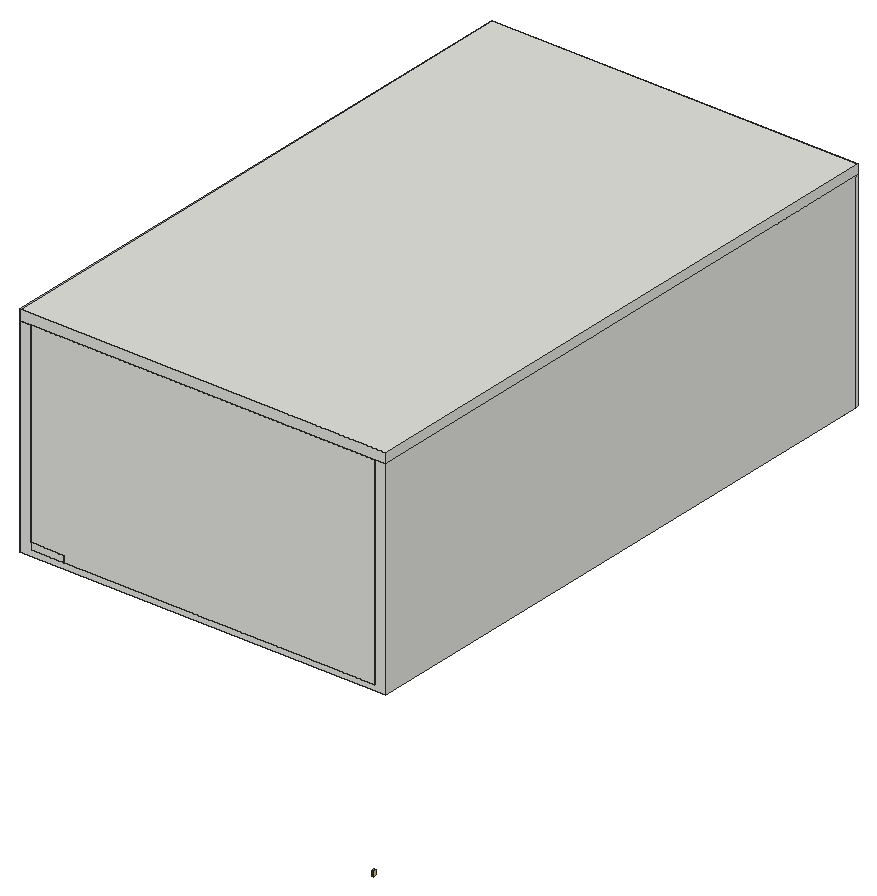
# SketchUp Ruby script. Lengths in inches.
U = 1.inch
M = Sketchup.active_model
def pt(a) = Geom::Point3d.new(a.map { |v| v * U })
def face(e, loops, mat)
  f = e.add_face(loops[0].map { |a| pt(a) })
  loops[1..].each { |l| e.add_face(l.map { |a| pt(a) }).erase! }
  f.material = f.back_material = mat if mat
  f
end
# faces: each face lists its corners as indices into pts; further lists are holes
def faces(e, pts, list, mat = nil) = list.each { |f| face(e, (f[0].is_a?(Array) ? f : [f]).map { |l| l.map { |i| pts[i] } }, mat) }
# xy, xz, yz: faces in a plane at the given z, y or x. An outline is a flat list of corners, or four numbers for a rectangle; further outlines are holes
def ring(l) = l.size == 4 ? [[l[0], l[1]], [l[2], l[1]], [l[2], l[3]], [l[0], l[3]]] : l.each_slice(2).to_a
def flat(e, list, mat, &to3) = list.each { |f| face(e, (f[0].is_a?(Array) ? f : [f]).map { |l| ring(l).map { |u, v| to3.(u, v) } }, mat) }
def xy(e, z, list, mat = nil) = flat(e, list, mat) { |x, y| [x, y, z] }
def xz(e, y, list, mat = nil) = flat(e, list, mat) { |x, z| [x, y, z] }
def yz(e, x, list, mat = nil) = flat(e, list, mat) { |y, z| [x, y, z] }
def lines(e, pts, list) = list.each { |a, b| e.add_line(pt(pts[a]), pt(pts[b])) }
# prism: a flat outline (further loops are holes) pulled along v
def prism(e, loops, v, mat = nil)
  f = face(e, loops, mat); d = Geom::Vector3d.new(v.map { |x| x * U })
  f.pushpull(f.normal.samedirection?(d) ? d.length : -d.length)
end
def box(e, o, s, mat = nil) = prism(e, [[o, [o[0] + s[0], o[1], o[2]], [o[0] + s[0], o[1] + s[1], o[2]], [o[0], o[1] + s[1], o[2]]]], [0, 0, s[2]], mat)
def at(x, y, z, deg = 0) = Geom::Transformation.translation(pt([x, y, z])) * Geom::Transformation.rotation(ORIGIN, Z_AXIS, deg.degrees)
def axes(o, x, y, z) = Geom::Transformation.new([*x, 0, *y, 0, *z, 0, *pt(o).to_a, 1])
def part(name) = M.definitions.add(name)
# library, detail: a bought-in or finely detailed component or shape, given as its bounding box
def library(name, o, s) = part(name).tap { |d| box(d.entities, o, s) }
def detail(e, o, s) = box(e.add_group.entities, o, s)
def put(e, d, t, mat = nil) = e.add_instance(d, t).tap { |i| i.material = mat if mat }
def group(e, t, mat = nil) = e.add_group.tap { |g| g.transformation = t; g.material = mat if mat }.entities
root = M.entities
M.materials.add("Material__1").color = [189, 132, 57]
M.materials.add("Material__10").color = [180, 24, 1]
M.materials.add("Material__2").color = [242, 239, 230]
M.materials.add("Material__3").color = [122, 114, 11]
M.materials.add("[0005_LightPink]").color = [206, 147, 156]
M.materials.add("[0007_MistyRose]").color = [255, 228, 225]
M.materials.add("[0011_Seashell]").color = [242, 232, 226]
M.materials.add("[0012_Bisque]").color = [255, 228, 196]
M.materials.add("[0021_DarkRed]").color = [58, 0, 0]
M.materials.add("[0022_Maroon]").color = [58, 0, 0]
M.materials.add("[0030_OldLace]").color = [253, 245, 230]
M.materials.add("[Color_000]").color = [255, 255, 255]
M.materials.add("[Color_004]").color = [142, 142, 142]
M.materials.add("[Tile Large Brown]").color = [193, 176, 158]
M.materials.add("cnwhc.com_草图联盟_1kmauOsh").color = [54, 52, 52]
M.materials.add("cnwhc.com_草图联盟_C8Y5Xp2O").color = [156, 156, 156]
M.materials["cnwhc.com_草图联盟_C8Y5Xp2O"].alpha = 0.15
M.materials.add("cnwhc.com_草图联盟_IHFcDxe1").color = [138, 151, 59]
M.materials.add("cnwhc.com_草图联盟_KNEfX85g").color = [162, 126, 87]
M.materials.add("cnwhc.com_草图联盟_QJow1Ky4").color = [144, 133, 65]
M.materials.add("cnwhc.com_草图联盟_z6N5x4Hv").color = [223, 205, 124]
c1 = library("JD\#1",[0,0,0],[1.32,0.83,0.01])
c2 = part("Untitled (20)")
xy(c2.entities,0,[[0,0,43.31,7.875],[43.31,0,47.24,7.875]],"[Color_000]")
xy(c2.entities,1.97,[[3.9375,0,43.31,3.15],[3.9375,3.15,23.62,4.72],[23.62,3.15,43.31,4.72],[3.9375,4.72,43.31,7.875]],"[Color_000]")
xy(c2.entities,3.9375,[[5.91,3.15,21.65,3.9375],[25.59,3.15,41.34,3.9375],[5.91,3.9375,21.65,4.72],[25.59,3.9375,41.34,4.72]],"[Color_000]")
xy(c2.entities,17.81,[[5.91,3.15,21.65,3.9375],[25.59,3.15,41.34,3.9375],[5.91,3.9375,21.65,4.72],[25.59,3.9375,41.34,4.72]],"[Color_000]")
xy(c2.entities,18.6,[[5.91,3.15,21.65,3.9375],[25.59,3.15,41.34,3.9375],[5.91,3.9375,21.65,4.72],[25.59,3.9375,41.34,4.72]],"[Color_000]")
xy(c2.entities,28.25,[[22.3,4.72,22.85,5.91],[24.27,4.72,24.8125,5.91]],"[Color_004]")
xy(c2.entities,29.04,[[22.3,4.72,22.85,5.51],[24.27,4.72,24.8125,5.51]],"[Color_004]")
xy(c2.entities,32.09,[[5.91,3.15,21.65,3.9375],[25.59,3.15,41.34,3.9375],[5.91,3.9375,21.65,4.72],[25.59,3.9375,41.34,4.72]],"[Color_000]")
xy(c2.entities,32.875,[[5.91,3.15,21.65,3.9375],[25.59,3.15,41.34,3.9375],[5.91,3.9375,21.65,4.72],[25.59,3.9375,41.34,4.72]],"[Color_000]")
xy(c2.entities,35.79,[[22.3,4.72,22.85,5.51],[24.27,4.72,24.8125,5.51]],"[Color_004]")
xy(c2.entities,36.58,[[22.3,4.72,22.85,5.91],[24.27,4.72,24.8125,5.91]],"[Color_004]")
xy(c2.entities,46.36,[[5.91,3.15,21.65,3.9375],[25.59,3.15,41.34,3.9375],[5.91,3.9375,21.65,4.72],[25.59,3.9375,41.34,4.72]],"[Color_000]")
xy(c2.entities,47.15,[[5.91,3.15,21.65,3.9375],[25.59,3.15,41.34,3.9375],[5.91,3.9375,21.65,4.72],[25.59,3.9375,41.34,4.72]],"[Color_000]")
xy(c2.entities,61.02,[[5.91,3.15,21.65,3.9375],[25.59,3.15,41.34,3.9375],[5.91,3.9375,21.65,4.72],[25.59,3.9375,41.34,4.72]],"[Color_000]")
xy(c2.entities,62.99,[[3.9375,0,43.31,3.15],[3.9375,3.15,23.62,4.72],[23.62,3.15,43.31,4.72],[3.9375,4.72,43.31,7.875]],"[Color_000]")
xy(c2.entities,66.93,[[0,0,47.24,7.875]],"[Color_000]")
xz(c2.entities,0,[[0,0,0,66.93,47.24,66.93,47.24,0,43.31,0,43.31,62.99,3.9375,62.99,3.9375,0],[3.9375,0,43.31,1.97]],"[Color_000]")
xz(c2.entities,3.15,[[[3.9375,1.97,23.62,62.99],[5.91,47.15,21.65,61.02],[5.91,3.9375,21.65,17.81],[5.91,18.6,21.65,32.09],[5.91,32.875,21.65,46.36]],[[23.62,1.97,43.31,62.99],[25.59,3.9375,41.34,17.81],[25.59,47.15,41.34,61.02],[25.59,18.6,41.34,32.09],[25.59,32.875,41.34,46.36]]],"[Color_000]")
xz(c2.entities,3.9375,[[5.91,3.9375,21.65,17.81],[25.59,3.9375,41.34,17.81],[5.91,18.6,21.65,32.09],[25.59,18.6,41.34,32.09],[5.91,32.875,21.65,46.36],
  [25.59,32.875,41.34,46.36],[5.91,47.15,21.65,61.02],[25.59,47.15,41.34,61.02]])
xz(c2.entities,4.72,[[[3.9375,1.97,23.62,62.99],[5.91,3.9375,21.65,17.81],[5.91,47.15,21.65,61.02],[5.91,18.6,21.65,32.09],[5.91,32.875,21.65,46.36]],[[23.62,1.97,43.31,62.99],[25.59,3.9375,41.34,17.81],[25.59,47.15,41.34,61.02],[25.59,18.6,41.34,32.09],[25.59,32.875,41.34,46.36]]],"[Color_000]")
xz(c2.entities,5.51,[[22.3,29.04,22.85,35.79],[24.27,29.04,24.8125,35.79]],"[Color_004]")
xz(c2.entities,5.91,[[22.3,28.25,22.85,36.58],[24.27,28.25,24.8125,36.58]],"[Color_004]")
xz(c2.entities,7.875,[[0,0,3.9375,0,3.9375,62.99,43.31,62.99,43.31,0,47.24,0,47.24,66.93,0,66.93],[3.9375,0,43.31,1.97]],"[Color_000]")
yz(c2.entities,0,[[0,0,7.875,66.93]],"[Color_000]")
yz(c2.entities,3.9375,[[0,1.97,3.15,62.99],[3.15,1.97,4.72,62.99],[4.72,1.97,7.875,62.99]],"[Color_000]")
yz(c2.entities,5.91,[[3.15,3.9375,3.9375,17.81],[3.9375,3.9375,4.72,17.81],[3.15,18.6,3.9375,32.09],[3.9375,18.6,4.72,32.09],[3.15,32.875,3.9375,46.36],
  [3.9375,32.875,4.72,46.36],[3.15,47.15,3.9375,61.02],[3.9375,47.15,4.72,61.02]],"[Color_000]")
yz(c2.entities,21.65,[[3.15,3.9375,3.9375,17.81],[3.9375,3.9375,4.72,17.81],[3.15,18.6,3.9375,32.09],[3.9375,18.6,4.72,32.09],[3.15,32.875,3.9375,46.36],
  [3.9375,32.875,4.72,46.36],[3.15,47.15,3.9375,61.02],[3.9375,47.15,4.72,61.02]],"[Color_000]")
yz(c2.entities,22.3,[[4.72,28.25,4.72,29.04,5.51,29.04,5.51,35.79,4.72,35.79,4.72,36.58,5.91,36.58,5.91,28.25]],"[Color_004]")
yz(c2.entities,22.85,[[4.72,28.25,5.91,28.25,5.91,36.58,4.72,36.58,4.72,35.79,5.51,35.79,5.51,29.04,4.72,29.04]],"[Color_004]")
yz(c2.entities,23.62,[[3.15,1.97,4.72,62.99]],"[Color_000]")
yz(c2.entities,24.27,[[4.72,28.25,4.72,29.04,5.51,29.04,5.51,35.79,4.72,35.79,4.72,36.58,5.91,36.58,5.91,28.25]],"[Color_004]")
yz(c2.entities,24.8125,[[4.72,28.25,5.91,28.25,5.91,36.58,4.72,36.58,4.72,35.79,5.51,35.79,5.51,29.04,4.72,29.04]],"[Color_004]")
yz(c2.entities,25.59,[[3.15,3.9375,3.9375,17.81],[3.9375,3.9375,4.72,17.81],[3.15,18.6,3.9375,32.09],[3.9375,18.6,4.72,32.09],[3.15,32.875,3.9375,46.36],
  [3.9375,32.875,4.72,46.36],[3.15,47.15,3.9375,61.02],[3.9375,47.15,4.72,61.02]],"[Color_000]")
yz(c2.entities,41.34,[[3.15,3.9375,3.9375,17.81],[3.9375,3.9375,4.72,17.81],[3.15,18.6,3.9375,32.09],[3.9375,18.6,4.72,32.09],[3.15,32.875,3.9375,46.36],
  [3.9375,32.875,4.72,46.36],[3.15,47.15,3.9375,61.02],[3.9375,47.15,4.72,61.02]],"[Color_000]")
yz(c2.entities,43.31,[[0,0,7.875,1.97],[0,1.97,3.15,62.99],[3.15,1.97,4.72,62.99],[4.72,1.97,7.875,62.99]],"[Color_000]")
yz(c2.entities,47.24,[[0,0,7.875,66.93]],"[Color_000]")
put(c2.entities,c1,axes([39.54,3.9375,4.43],[1,0,0],[0,0,1],[0,-1,0]))
put(c2.entities,c1,axes([19.85,3.9375,4.43],[1,0,0],[0,0,1],[0,-1,0]))
c3 = library("B36CD50SNS_tradeCAD",[0,0,0],[35.84,30.35,69.65])
c4 = library("Oven",[-9.26,-22.59,0.07],[23.42,23.91,23.21])
c5 = library("ZSA1202RSS",[0,0,0],[29.9375,17.9,16.4375])
c6 = library("switch+board",[0,0,0],[0.88,10.49,5.27])
c7 = library("Grupo3\#1",[-2.41,-4.18,0],[4.82,8.16,14.49])
c8 = library("Group\#35",[-453.95,-270.9,-0.08],[243.89,243.63,216.82])
c9 = library("Group\#42",[118.34,-437.05,68.8],[33.09,42.97,27.32])
c10 = library("Group\#43",[91.875,-459.8125,1.36],[84.84,84.82,167.94])
c11 = library("Group\#44",[93.63,-458.06,3.28],[81.33,81.31,90.04])
c12 = library("Group\#45",[114.46,-437.1875,150.05],[39.68,39.57,39.67])
c13 = library("Group\#46",[177.52,-496.26,3.28],[81.21,81.23,127.94])
c14 = library("Group\#47",[175.77,-498.01,1.36],[84.71,84.74,167.94])
c15 = library("Group\#48",[198.24,-475.92,149.53],[39.78,40.55,40.71])
c16 = library("Group\#49",[-248.47,-468.28,0.39],[392.05,393.05,278.56])
c17 = library("Group\#50",[-141.57,-278.65,11.2],[96.36,96.33,131.41])
c18 = library("Group\#51",[-62.08,-202.43,11.2],[96.04,96.07,131.41])
c19 = library("Group\#52",[18.13,-280.93,11.2],[96.51,96.54,131.41])
c20 = library("Group\#53",[-213.25,-366.61,11.2],[96.18,96.15,131.41])
c21 = library("Group\#54",[-61.03,-358.93,11.2],[96.54,96.51,131.41])
c22 = library("Group\#55",[8.05,-292.87,22.71],[116.19,111.01,218.49])
c23 = library("Group\#56",[-64.85,-368.89,23],[127.95,108.9,222.0625])
c24 = library("Group\#57",[-143.92,-281.53,22.82],[119.68,105.06,218.38])
c25 = library("Group\#58",[-64.19,-232.55,22.9],[102.65,128.29,224.14])
c26 = library("Group\#59",[-225.25,-376.69,19.19],[116.52,116.69,261.73])
c27 = library("Group\#60",[-138.35,-437.94,11.2],[96.49,96.52,131.41])
c28 = library("Group\#61",[-142.58,-458.38,19.87],[79.66,135.74,256])
c29 = part("KITCHEN+ITEMS+(37)")
put(c29.entities,c8,at(0,0,0))
put(c29.entities,c9,at(0,0,0),"cnwhc.com_草图联盟_IHFcDxe1")
put(c29.entities,c10,at(0,0,0),"cnwhc.com_草图联盟_C8Y5Xp2O")
put(c29.entities,c11,at(0,0,0),"cnwhc.com_草图联盟_QJow1Ky4")
put(c29.entities,c12,at(0,0,0),"cnwhc.com_草图联盟_KNEfX85g")
put(c29.entities,c13,at(0,0,0),"cnwhc.com_草图联盟_z6N5x4Hv")
put(c29.entities,c14,at(0,0,0),"cnwhc.com_草图联盟_C8Y5Xp2O")
put(c29.entities,c15,at(0,0,0),"cnwhc.com_草图联盟_KNEfX85g")
put(c29.entities,c16,at(0,0,0),"cnwhc.com_草图联盟_1kmauOsh")
put(c29.entities,c17,at(0,0,0),"cnwhc.com_草图联盟_C8Y5Xp2O")
put(c29.entities,c18,at(0,0,0),"cnwhc.com_草图联盟_C8Y5Xp2O")
put(c29.entities,c19,at(0,0,0),"cnwhc.com_草图联盟_C8Y5Xp2O")
put(c29.entities,c20,at(0,0,0),"cnwhc.com_草图联盟_C8Y5Xp2O")
put(c29.entities,c21,at(0,0,0),"cnwhc.com_草图联盟_C8Y5Xp2O")
put(c29.entities,c22,at(0,0,0),"cnwhc.com_草图联盟_1kmauOsh")
put(c29.entities,c23,at(0,0,0),"cnwhc.com_草图联盟_1kmauOsh")
put(c29.entities,c24,at(0,0,0),"cnwhc.com_草图联盟_1kmauOsh")
put(c29.entities,c25,at(0,0,0),"cnwhc.com_草图联盟_1kmauOsh")
put(c29.entities,c26,at(0,0,0))
put(c29.entities,c27,at(0,0,0),"cnwhc.com_草图联盟_C8Y5Xp2O")
put(c29.entities,c28,at(0,0,0))
c30 = library("C_HOB",[0,0,0],[30.71,17.32,2.28])
c31 = library("Component_12",[0,0,0],[17.72,31.5,20.63])
c32 = library("secto_design_octo_lamp_150sm",[-45.69,-78.93,-193.9375],[1.18,1.52,2.78])
c33 = library("Untitled",[-2.37,-2.84,0],[34.77,46.37,39.61])
c34 = library("Group\#13",[70.57,7290.35,1177],[106.36,95.58,107.8])
c35 = library("Group\#14",[99.22,7286.02,1075.87],[101.63,96.21,134.31])
c36 = library("Group\#12",[73.8125,7223.02,1078.11],[130.55,102.07,69.6])
c37 = library("Group\#11",[51.66,7209.26,1075.25],[220.83,167.48,13.5625])
c38 = library("Group\#15",[141.6875,7219.59,1077.95],[111.05,77.92,100.97])
c39 = library("Group\#16",[180.93,7251.18,1124.56],[65.88,104.93,74.66])
c40 = library("Group\#39",[0,0,0],[35.16,49.83,62.5625])
xy(root,0,[[1.875,0,219.125,349.0625],[1.875,349.0625,219.125,350.4375]])
xy(root,3.25,[[27.875,0,212.75,0,212.75,344.4375,174.95,344.4375,174.95,324.4375,27.875,324.4375]],"[Tile Large Brown]")
xy(root,5.25,[[120.66,320.4375,121.78,324.4375],[174.04,320.4375,174.95,324.4375],[121.78,324.4375,174.04,342.4375]])
xy(root,7.25,[[7.875,0,27.875,206.4375],[7.875,206.4375,27.875,344.4375],[27.875,206.4375,27.875,324.4375,31.875,324.4375,31.875,305.07,31.75,305.07,31.75,304.77,31.875,304.77,31.875,285.4,31.75,285.4,31.75,285.1,31.875,285.1,31.875,265.74,31.57,265.74,31.57,265.4375,31.875,265.4375,31.875,246.07,31.57,246.07,31.57,245.77,31.875,245.77,31.875,226.4,31.57,226.4,31.57,226.1,31.875,226.1,31.875,206.4375],[31.875,320.4375,92.74,324.4375],[92.74,320.4375,120.66,324.4375],
  [27.875,324.4375,31.875,344.4375],[31.875,324.4375,92.74,344.4375]])
xy(root,21.0625,[[12.6,212.83,26.79,237.4]])
xy(root,23.61,[[94.18,320.4375,119.93,342.4375]])
xy(root,30.1875,[[[7.875,206.4375,7.875,344.4375,31.875,344.4375,31.875,305.07,31.75,305.07,31.75,304.77,31.875,304.77,31.875,285.4,31.75,285.4,31.75,285.1,31.875,285.1,31.875,265.74,31.57,265.74,31.57,265.4375,31.875,265.4375,31.875,246.07,31.57,246.07,31.57,245.77,31.875,245.77,31.875,226.4,31.57,226.4,31.57,226.1,31.875,226.1,31.875,206.4375],[12.6,212.83,26.79,237.4]],[31.875,320.4375,92.74,344.4375]])
xy(root,31.25,[[[7.875,206.4375,31.875,206.4375,31.875,226.1,31.57,226.1,31.57,226.4,31.875,226.4,31.875,245.77,31.57,245.77,31.57,246.07,31.875,246.07,31.875,265.4375,31.57,265.4375,31.57,265.74,31.875,265.74,31.875,285.1,31.75,285.1,31.75,285.4,31.875,285.4,31.875,304.77,31.75,304.77,31.75,305.07,31.875,305.07,31.875,344.4375,7.875,344.4375],[12.6,212.83,26.79,237.4]],[31.875,320.4375,92.74,344.4375]])
xy(root,39.25,[[1.875,241.12,7.875,291.68]])
xy(root,43.3,[[94.18,320.4375,119.93,342.4375]])
xy(root,43.97,[[94.18,320.4375,119.93,342.4375]])
xy(root,54.5,[[7.875,291.68,7.875,344.4375,92.74,344.4375,92.74,324.4375,68.82,324.4375,68.82,324.875,68.52,324.875,68.52,324.4375,48.35,324.4375,48.35,324.875,48.05,324.875,48.05,324.4375,27.875,324.4375,27.875,291.68]])
xy(root,55.25,[[7.875,291.68,27.875,291.68,27.875,324.4375,48.05,324.4375,48.05,324.875,48.35,324.875,48.35,324.4375,68.52,324.4375,68.52,324.875,68.82,324.875,68.82,324.4375,92.74,324.4375,92.74,344.4375,7.875,344.4375]])
xy(root,55.84,[[7.875,292.27,27.875,310.77]])
xy(root,56.48,[[94.18,320.4375,119.93,342.4375]])
xy(root,56.96,[[93.75,320.4375,120.66,320.5625]])
xy(root,57.46,[[94.25,320.4375,120.16,320.5625]])
xy(root,64.125,[[121.78,320.4375,147.91,342.4375],[147.91,320.4375,148.29,342.4375],[148.29,320.4375,172.91,342.4375],[172.91,320.4375,174.04,342.4375]])
xy(root,64.4375,[[121.78,320.4375,147.91,320.5625],[147.91,320.4375,148.29,320.5625],[148.29,320.4375,172.91,320.5625],[172.91,320.4375,174.04,320.5625]])
xy(root,64.71,[[122.0625,320.4375,147.63,320.5625],[148.5625,320.4375,172.91,320.5625],[172.91,320.4375,173.76,320.5625]])
xy(root,66.96,[[7.875,292.27,27.875,310.77]])
xy(root,67.65,[[7.875,292.27,27.875,310.77]])
xy(root,77.82,[[94.25,320.4375,120.16,320.5625]])
xy(root,78.04,[[122.0625,320.4375,147.63,320.5625],[148.5625,320.4375,173.76,320.5625]])
xy(root,78.09,[[7.875,292.27,27.875,310.77]])
xy(root,78.3125,[[93.75,320.4375,120.66,320.5625],[121.78,320.4375,147.91,320.5625],[147.91,320.4375,148.29,320.5625],[148.29,320.4375,174.04,320.5625]])
xy(root,78.75,[[7.875,291.68,27.875,318.0625],[7.875,318.0625,27.875,324.4375],[92.74,320.4375,174.95,320.4375,174.95,344.4375,169.83,344.4375,169.83,324.4375,149.85,324.4375,149.85,324.5625,149.55,324.5625,149.55,324.4375,129.57,324.4375,129.57,324.5625,129.27,324.5625,129.27,324.4375,109.29,324.4375,109.29,324.5625,108.99,324.5625,108.99,324.4375,92.74,324.4375],[7.875,324.4375,27.875,344.4375],[27.875,324.4375,36.16,344.4375],
  [36.16,324.4375,36.16,344.4375,64.45,344.4375,64.45,324.4375,48.35,324.4375,48.35,324.875,48.05,324.875,48.05,324.4375],[48.05,324.4375,48.35,324.875],[64.45,324.4375,64.45,344.4375,92.74,344.4375,92.74,324.4375,68.82,324.4375,68.82,324.875,68.52,324.875,68.52,324.4375],[68.52,324.4375,68.82,324.875]])
xy(root,78.75,[[7.875,206.4375,27.875,291.68]],"[0007_MistyRose]")
xy(root,79.25,[[7.875,206.4375,27.875,206.4375,27.875,226.1,27.75,226.1,27.75,226.4,27.875,226.4,27.875,241.12,7.875,241.12],[27.75,226.1,27.875,226.4],[1.875,241.12,7.875,291.68],[7.875,241.12,27.875,241.12,27.875,245.77,27.75,245.77,27.75,246.07,27.875,246.07,27.875,265.4375,27.75,265.4375,27.75,265.74,27.875,265.74,27.875,285.1,27.75,285.1,27.75,285.4,27.875,285.4,27.875,291.68,7.875,291.68],[27.75,245.77,27.875,246.07],
  [27.75,265.4375,27.875,265.74],[27.75,285.1,27.875,285.4],[7.875,291.68,27.875,291.68,27.875,304.77,27.75,304.77,27.75,305.07,27.875,305.07,27.875,324.4375,7.875,324.4375],[27.75,304.77,27.875,305.07],[7.875,324.4375,48.15,324.4375,48.15,324.5625,48.45,324.5625,48.45,324.4375,68.43,324.4375,68.43,324.5625,68.73,324.5625,68.73,324.4375,88.71,324.4375,88.71,324.5625,89.01,324.5625,89.01,324.4375,92.74,324.4375,92.74,344.4375,7.875,344.4375],
  [48.15,324.4375,48.45,324.5625],[68.43,324.4375,68.73,324.5625],[88.71,324.4375,89.01,324.5625],[92.74,324.4375,92.74,344.4375,169.83,344.4375,169.83,324.4375,149.85,324.4375,149.85,324.5625,149.55,324.5625,149.55,324.4375,129.57,324.4375,129.57,324.5625,129.27,324.5625,129.27,324.4375,109.29,324.4375,109.29,324.5625,108.99,324.5625,108.99,324.4375]])
xy(root,123.25,[[1.875,0,1.875,349.0625,219.125,349.0625,219.125,0,212.75,0,212.75,344.4375,7.875,344.4375,7.875,0],[7.875,0,27.875,206.4375],[7.875,206.4375,7.875,324.4375,27.875,324.4375,27.875,305.07,27.75,305.07,27.75,304.77,27.875,304.77,27.875,285.4,27.75,285.4,27.75,285.1,27.875,285.1,27.875,265.74,27.75,265.74,27.75,265.4375,27.875,265.4375,27.875,246.07,27.75,246.07,27.75,245.77,27.875,245.77,27.875,226.4,27.75,226.4,27.75,226.1,27.875,226.1,27.875,206.4375],[7.875,324.4375,7.875,344.4375,169.83,344.4375,169.83,324.4375,149.85,324.4375,149.85,324.5625,149.55,324.5625,149.55,324.4375,129.57,324.4375,129.57,324.5625,129.27,324.5625,129.27,324.4375,109.29,324.4375,109.29,324.5625,108.99,324.5625,108.99,324.4375,89.01,324.4375,89.01,324.5625,88.71,324.5625,88.71,324.4375,68.73,324.4375,68.73,324.5625,68.43,324.5625,68.43,324.4375,48.45,324.4375,48.45,324.5625,48.15,324.5625,48.15,324.4375],[1.875,349.0625,219.125,350.4375]])
xy(root,123.25,[[[95.39,234.92,146.73,296.17],[123.59,242.42,125.03,242.53,126.45,242.79,127.84,243.2,129.17,243.75,130.44,244.44,131.64,245.26,132.74,246.2,133.73,247.25,134.61,248.39,135.37,249.625,135.99,250.93,136.48,252.29,136.8125,253.7,137,255.13,137.04,256.58,136.93,258.02,136.67,259.4375,136.26,260.83,135.71,262.16,135.02,263.43,134.2,264.625,133.26,265.73,132.21,266.72,131.07,267.6,129.83,268.36,128.53,268.98,127.17,269.46,125.76,269.8,124.33,269.99,122.88,270.03,121.44,269.92,120.02,269.66,118.63,269.25,117.3,268.69,116.03,268.01,114.83,267.1875,113.73,266.25,112.74,265.2,111.86,264.05,111.1,262.82,110.48,261.52,109.99,260.15,109.65,258.75,109.47,257.32,109.43,255.87,109.54,254.43,109.8,253.01,110.21,251.62,110.76,250.29,111.45,249.01,112.27,247.82,113.21,246.72,114.26,245.73,115.4,244.85,116.64,244.09,117.94,243.47,119.3,242.98,120.71,242.64,122.14,242.45]]],"[0005_LightPink]")
xy(root,123.25,[[123.59,242.42,122.14,242.45,120.71,242.64,119.3,242.98,117.94,243.47,116.64,244.09,115.4,244.85,114.26,245.73,113.21,246.72,112.27,247.82,111.45,249.01,110.76,250.29,110.21,251.62,109.8,253.01,109.54,254.43,109.43,255.87,109.47,257.32,109.65,258.75,109.99,260.15,110.48,261.52,111.1,262.82,111.86,264.05,112.74,265.2,113.73,266.25,114.83,267.1875,116.03,268.01,117.3,268.69,118.63,269.25,120.02,269.66,121.44,269.92,122.88,270.03,124.33,269.99,125.76,269.8,127.17,269.46,128.53,268.98,129.83,268.36,131.07,267.6,132.21,266.72,133.26,265.73,134.2,264.625,135.02,263.43,135.71,262.16,136.26,260.83,136.67,259.4375,136.93,258.02,137.04,256.58,137,255.13,136.8125,253.7,136.48,252.29,135.99,250.93,135.37,249.625,134.61,248.39,133.73,247.25,132.74,246.2,131.64,245.26,130.44,244.44,129.17,243.75,127.84,243.2,126.45,242.79,125.03,242.53]],"[0022_Maroon]")
xy(root,123.25,[[[27.875,0,27.875,226.1,27.75,226.1,27.75,226.4,27.875,226.4,27.875,245.77,27.75,245.77,27.75,246.07,27.875,246.07,27.875,265.4375,27.75,265.4375,27.75,265.74,27.875,265.74,27.875,285.1,27.75,285.1,27.75,285.4,27.875,285.4,27.875,304.77,27.75,304.77,27.75,305.07,27.875,305.07,27.875,324.4375,48.15,324.4375,48.15,324.5625,48.45,324.5625,48.45,324.4375,68.43,324.4375,68.43,324.5625,68.73,324.5625,68.73,324.4375,88.71,324.4375,88.71,324.5625,89.01,324.5625,89.01,324.4375,108.99,324.4375,108.99,324.5625,109.29,324.5625,109.29,324.4375,129.27,324.4375,129.27,324.5625,129.57,324.5625,129.57,324.4375,149.55,324.4375,149.55,324.5625,149.85,324.5625,149.85,324.4375,169.83,324.4375,169.83,344.4375,212.75,344.4375,212.75,0],[35.81,218.1,202.93,312.98]]],"[0030_OldLace]")
xy(root,127.5625,[[[35.81,218.1,202.93,312.98],[95.39,234.92,146.73,296.17]]],"[0030_OldLace]")
xy(root,129.25,[[1.875,0,219.125,350.4375]])
xz(root,0,[[1.875,0,219.125,0,219.125,123.25,212.75,123.25,212.75,3.25,7.875,3.25,7.875,123.25,1.875,123.25],[27.875,3.25,212.75,3.25,212.75,123.25,7.875,123.25,7.875,7.25,27.875,7.25],[7.875,3.25,27.875,7.25],[1.875,123.25,219.125,129.25]])
xz(root,206.4375,[[7.875,30.1875,31.875,31.25],[7.875,78.75,27.875,79.25]])
xz(root,206.4375,[[7.875,79.25,27.875,123.25]],"[0007_MistyRose]")
xz(root,206.4375,[[7.875,7.25,31.875,30.1875]],"[0011_Seashell]")
xz(root,212.83,[[12.6,21.0625,26.79,30.1875],[12.6,30.1875,26.79,31.25]])
xz(root,218.1,[[35.81,123.25,202.93,127.5625]])
xz(root,226.1,[[31.57,7.25,31.875,30.1875],[31.57,30.1875,31.875,31.25],[27.75,79.25,27.875,123.25]])
xz(root,226.4,[[31.57,7.25,31.875,30.1875],[31.57,30.1875,31.875,31.25],[27.75,79.25,27.875,123.25]])
xz(root,234.92,[[95.39,123.25,146.73,127.5625]],"[0030_OldLace]")
xz(root,237.4,[[12.6,21.0625,26.79,30.1875],[12.6,30.1875,26.79,31.25]])
xz(root,241.12,[[1.875,39.25,7.875,79.25]])
xz(root,245.77,[[31.57,7.25,31.875,30.1875],[31.57,30.1875,31.875,31.25],[27.75,79.25,27.875,123.25]])
xz(root,246.07,[[31.57,7.25,31.875,30.1875],[31.57,30.1875,31.875,31.25],[27.75,79.25,27.875,123.25]])
xz(root,265.4375,[[31.57,7.25,31.875,30.1875],[31.57,30.1875,31.875,31.25],[27.75,79.25,27.875,123.25]])
xz(root,265.74,[[31.57,7.25,31.875,30.1875],[31.57,30.1875,31.875,31.25],[27.75,79.25,27.875,123.25]])
xz(root,285.1,[[31.75,7.25,31.875,30.1875],[31.75,30.1875,31.875,31.25],[27.75,79.25,27.875,123.25]])
xz(root,285.4,[[31.75,7.25,31.875,30.1875],[31.75,30.1875,31.875,31.25],[27.75,79.25,27.875,123.25]])
xz(root,291.68,[[7.875,54.5,27.875,55.25]])
xz(root,291.68,[[1.875,39.25,7.875,39.25,7.875,55.25,27.875,55.25,27.875,78.75,7.875,78.75,7.875,79.25,1.875,79.25]],"[0007_MistyRose]")
xz(root,292.27,[[7.875,55.84,27.875,66.96],[7.875,66.96,27.875,67.65],[7.875,67.65,27.875,78.09]])
xz(root,296.17,[[95.39,123.25,146.73,127.5625]])
xz(root,304.77,[[31.75,7.25,31.875,30.1875],[31.75,30.1875,31.875,31.25],[27.75,79.25,27.875,123.25]])
xz(root,305.07,[[31.75,7.25,31.875,30.1875],[31.75,30.1875,31.875,31.25],[27.75,79.25,27.875,123.25]])
xz(root,310.77,[[7.875,66.96,27.875,67.65]])
xz(root,310.77,[[7.875,55.84,27.875,66.96],[7.875,67.65,27.875,78.09]],"[0007_MistyRose]")
xz(root,312.98,[[35.81,123.25,202.93,127.5625]],"[0030_OldLace]")
xz(root,320.4375,[[62.31,7.25,62.61,30.1875],[94.18,43.3,119.93,43.97],[121.78,64.125,174.04,64.4375]])
xz(root,320.4375,[[120.66,5.25,121.78,65.56],[174.04,5.25,174.95,78.3125],[31.875,7.25,62.31,30.1875],[62.61,7.25,92.74,30.1875],[92.74,7.25,93.75,7.25,93.75,78.3125,174.04,78.3125,174.04,78.75,92.74,78.75],
  [[93.75,7.25,120.66,56.96],[94.18,23.61,119.93,56.48]],[120.66,65.56,121.78,78.3125],[174.04,78.3125,174.95,78.75]],"[0005_LightPink]")
xz(root,320.4375,[[94.25,57.46,120.16,77.82],[122.0625,64.71,147.63,78.04],[148.5625,64.71,173.76,78.04]],"[0007_MistyRose]")
xz(root,320.4375,[[31.875,30.1875,62.31,31.25],[62.31,30.1875,62.61,31.25],[62.61,30.1875,92.74,31.25]],"[0021_DarkRed]")
xz(root,320.5625,[[[93.75,56.96,120.66,78.3125],[94.25,57.46,120.16,77.82]],[[121.78,64.4375,147.91,78.3125],[122.0625,64.71,147.63,78.04]],[147.91,64.4375,148.29,78.3125],[[148.29,64.4375,174.04,78.3125],[148.5625,64.71,173.76,78.04]]])
xz(root,324.4375,[[7.875,78.75,27.875,79.25],[7.875,79.25,27.875,123.25]])
xz(root,324.4375,[[27.875,79.25,48.15,123.25],[48.45,79.25,68.43,123.25],[68.73,79.25,88.71,123.25],[89.01,79.25,108.99,123.25],[109.29,79.25,129.27,123.25],
  [129.57,79.25,149.55,123.25],[149.85,79.25,169.83,123.25]],"[0005_LightPink]")
xz(root,324.4375,[[27.875,55.25,48.05,78.75],[48.35,55.25,68.52,78.75],[68.82,55.25,92.74,78.75]],"[0007_MistyRose]")
xz(root,324.4375,[[27.875,3.25,174.95,3.25,174.95,5.25,120.66,5.25,120.66,7.25,27.875,7.25]],"[0012_Bisque]")
xz(root,324.4375,[[27.875,54.5,48.05,55.25],[48.35,54.5,68.52,55.25],[68.82,54.5,92.74,55.25],[27.875,78.75,108.99,79.25],[109.29,78.75,129.27,79.25],
  [129.57,78.75,149.55,79.25],[149.85,78.75,169.83,79.25]],"[0021_DarkRed]")
xz(root,324.5625,[[48.15,79.25,48.45,123.25],[68.43,79.25,68.73,123.25],[88.71,79.25,89.01,123.25],[108.99,79.25,109.29,123.25],[129.27,79.25,129.57,123.25],
  [149.55,79.25,149.85,123.25]])
xz(root,324.5625,[[108.99,78.75,109.29,79.25],[129.27,78.75,129.57,79.25],[149.55,78.75,149.85,79.25]],"[0021_DarkRed]")
xz(root,324.875,[[48.05,54.5,48.35,55.25],[68.52,54.5,68.82,55.25],[48.05,55.25,48.35,78.75],[68.52,55.25,68.82,78.75]])
xz(root,342.4375,[[121.78,5.25,174.04,64.125],[94.18,23.61,119.93,43.3],[94.18,43.97,119.93,56.48]])
xz(root,344.4375,[[174.95,3.25,212.75,3.25,212.75,123.25,169.83,123.25,169.83,78.75,174.95,78.75],[7.875,7.25,31.875,30.1875],[31.875,7.25,92.74,30.1875],[92.74,7.25,92.74,79.25,169.83,79.25,169.83,78.75,174.95,78.75,174.95,7.25],[7.875,30.1875,31.875,31.25],
  [31.875,30.1875,92.74,31.25],[7.875,31.25,92.74,54.5],[7.875,54.5,92.74,55.25],[7.875,78.75,92.74,79.25],[7.875,79.25,169.83,123.25]])
xz(root,349.0625,[[1.875,0,219.125,123.25]])
xz(root,350.4375,[[1.875,0,219.125,123.25],[1.875,123.25,219.125,129.25]])
yz(root,1.875,[[[0,0,349.0625,123.25],[241.12,39.25,291.68,79.25]],[349.0625,0,350.4375,123.25],[0,123.25,350.4375,129.25]])
yz(root,7.875,[[0,7.25,206.4375,30.1875],[206.4375,7.25,344.4375,30.1875],[0,30.1875,206.4375,31.25],[206.4375,30.1875,344.4375,31.25],[0,31.25,344.4375,31.25,344.4375,54.5,291.68,54.5,291.68,39.25,241.12,39.25,241.12,78.75,0,78.75],
  [291.68,54.5,344.4375,55.25],[292.27,55.84,310.77,66.96],[292.27,66.96,310.77,67.65],[292.27,67.65,310.77,78.09],[0,78.75,206.4375,79.25],
  [206.4375,78.75,241.12,79.25],[241.12,78.75,291.68,79.25],[291.68,78.75,324.4375,79.25],[324.4375,78.75,344.4375,79.25],[0,79.25,206.4375,123.25],
  [206.4375,79.25,324.4375,123.25],[324.4375,79.25,344.4375,123.25]])
yz(root,12.6,[[212.83,21.0625,237.4,30.1875],[212.83,30.1875,237.4,31.25]])
yz(root,26.79,[[212.83,21.0625,237.4,30.1875],[212.83,30.1875,237.4,31.25]])
yz(root,27.75,[[226.1,79.25,226.4,123.25],[245.77,79.25,246.07,123.25],[265.4375,79.25,265.74,123.25],[285.1,79.25,285.4,123.25],[304.77,79.25,305.07,123.25]])
yz(root,27.875,[[292.27,66.96,310.77,67.65]])
yz(root,27.875,[[206.4375,79.25,226.1,123.25],[226.4,79.25,245.77,123.25],[246.07,79.25,265.4375,123.25],[265.74,79.25,285.1,123.25],[285.4,79.25,304.77,123.25],
  [305.07,79.25,324.4375,123.25]],"[0005_LightPink]")
yz(root,27.875,[[[291.68,55.25,324.4375,78.75],[292.27,55.84,310.77,78.09]]],"[0007_MistyRose]")
yz(root,27.875,[[0,3.25,324.4375,7.25]],"[0012_Bisque]")
yz(root,27.875,[[291.68,54.5,324.4375,55.25],[206.4375,78.75,324.4375,79.25]],"[0021_DarkRed]")
yz(root,31.57,[[226.1,7.25,226.4,30.1875],[245.77,7.25,246.07,30.1875],[265.4375,7.25,265.74,30.1875],[226.1,30.1875,226.4,31.25],[245.77,30.1875,246.07,31.25],
  [265.4375,30.1875,265.74,31.25]])
yz(root,31.75,[[285.1,7.25,285.4,30.1875],[304.77,7.25,305.07,30.1875],[285.1,30.1875,285.4,31.25],[304.77,30.1875,305.07,31.25]])
yz(root,31.875,[[320.4375,7.25,324.4375,30.1875],[324.4375,7.25,344.4375,30.1875],[320.4375,30.1875,324.4375,31.25],[324.4375,30.1875,344.4375,31.25]])
yz(root,31.875,[[206.4375,7.25,226.1,30.1875],[226.4,7.25,245.77,30.1875],[246.07,7.25,265.4375,30.1875],[265.74,7.25,285.1,30.1875],[285.4,7.25,304.77,30.1875],
  [305.07,7.25,320.4375,30.1875]],"[0005_LightPink]")
yz(root,31.875,[[206.4375,30.1875,226.1,31.25],[226.4,30.1875,245.77,31.25],[246.07,30.1875,265.4375,31.25],[265.74,30.1875,285.1,31.25],[285.4,30.1875,304.77,31.25],
  [305.07,30.1875,320.4375,31.25]],"[0021_DarkRed]")
yz(root,35.81,[[218.1,123.25,312.98,127.5625]],"[0030_OldLace]")
yz(root,48.05,[[324.4375,54.5,324.875,55.25],[324.4375,55.25,324.875,78.75]])
yz(root,48.15,[[324.4375,79.25,324.5625,123.25]])
yz(root,48.35,[[324.4375,54.5,324.875,55.25],[324.4375,55.25,324.875,78.75]])
yz(root,48.45,[[324.4375,79.25,324.5625,123.25]])
yz(root,68.43,[[324.4375,79.25,324.5625,123.25]])
yz(root,68.52,[[324.4375,54.5,324.875,55.25],[324.4375,55.25,324.875,78.75]])
yz(root,68.73,[[324.4375,79.25,324.5625,123.25]])
yz(root,68.82,[[324.4375,54.5,324.875,55.25],[324.4375,55.25,324.875,78.75]])
yz(root,88.71,[[324.4375,79.25,324.5625,123.25]])
yz(root,89.01,[[324.4375,79.25,324.5625,123.25]])
yz(root,92.74,[[320.4375,7.25,344.4375,30.1875],[320.4375,30.1875,344.4375,31.25],[320.4375,31.25,320.4375,78.75,324.4375,78.75,324.4375,54.5,344.4375,54.5,344.4375,31.25],[324.4375,54.5,344.4375,55.25],[324.4375,55.25,344.4375,78.75]])
yz(root,93.75,[[320.4375,56.96,320.5625,78.3125]])
yz(root,94.18,[[320.4375,23.61,342.4375,43.3],[320.4375,43.97,342.4375,56.48]])
yz(root,94.25,[[320.4375,57.46,320.5625,77.82]])
yz(root,95.39,[[234.92,123.25,296.17,127.5625]],"[0030_OldLace]")
yz(root,108.99,[[324.4375,78.75,324.5625,79.25],[324.4375,79.25,324.5625,123.25]])
yz(root,109.29,[[324.4375,78.75,324.5625,79.25],[324.4375,79.25,324.5625,123.25]])
yz(root,119.93,[[320.4375,23.61,342.4375,43.3],[320.4375,43.97,342.4375,56.48]])
yz(root,120.16,[[320.4375,57.46,320.5625,65.56],[320.4375,65.56,320.5625,77.82]])
yz(root,120.66,[[320.4375,5.25,324.4375,7.25],[320.4375,56.96,320.5625,65.56],[320.4375,65.56,320.5625,78.3125]])
yz(root,121.78,[[320.4375,5.25,342.4375,64.125],[320.4375,64.4375,320.5625,65.56],[320.4375,65.56,320.5625,78.3125]])
yz(root,122.0625,[[320.4375,64.71,320.5625,65.56],[320.4375,65.56,320.5625,78.04]])
yz(root,129.27,[[324.4375,78.75,324.5625,79.25],[324.4375,79.25,324.5625,123.25]])
yz(root,129.57,[[324.4375,78.75,324.5625,79.25],[324.4375,79.25,324.5625,123.25]])
yz(root,146.73,[[234.92,123.25,296.17,127.5625]],"[0030_OldLace]")
yz(root,147.63,[[320.4375,64.71,320.5625,65.56],[320.4375,65.56,320.5625,78.04]])
yz(root,148.5625,[[320.4375,64.71,320.5625,65.56],[320.4375,65.56,320.5625,78.04]])
yz(root,149.55,[[324.4375,78.75,324.5625,79.25],[324.4375,79.25,324.5625,123.25]])
yz(root,149.85,[[324.4375,78.75,324.5625,79.25],[324.4375,79.25,324.5625,123.25]])
yz(root,169.83,[[324.4375,78.75,344.4375,79.25],[324.4375,79.25,344.4375,123.25]])
yz(root,173.76,[[320.4375,64.71,320.5625,65.56],[320.4375,65.56,320.5625,78.04]])
yz(root,174.04,[[320.4375,5.25,342.4375,64.125],[320.4375,64.4375,320.5625,65.56],[320.4375,65.56,320.5625,78.3125]])
yz(root,174.95,[[324.4375,3.25,344.4375,7.25],[320.4375,5.25,324.4375,5.25,324.4375,7.25,344.4375,7.25,344.4375,31.25,320.4375,31.25],[320.4375,31.25,344.4375,55.25],[320.4375,55.25,344.4375,78.75]])
yz(root,202.93,[[218.1,123.25,312.98,127.5625]],"[0030_OldLace]")
yz(root,212.75,[[0,3.25,344.4375,123.25]])
yz(root,219.125,[[0,0,349.0625,123.25],[349.0625,0,350.4375,123.25],[0,123.25,350.4375,129.25]])
p = [[174.95,325.22,78.73],[174.95,324.4375,78.75],[426.43,-11208.82,0],[427.43,-11208.82,0],[427.43,-11207.82,0]]
lines(root,p,[[0,1],[2,3],[3,4],[4,2]])
put(root,c2,axes([0,291.68,39.25],[0,-1.07,0],[1,0,0],[0,0,0.61]),"[0007_MistyRose]")
put(root,c3,axes([121.65,318.3125,4.63],[1.45791,0,0],[0,1,0],[0,0,0.85598]))
put(root,c4,axes([104.54,340.93,23.55],[1.08659,0,0],[0,1,0],[0,0,0.84959]))
put(root,c5,axes([93.75,317.83,43.99],[0.87436,0,0],[0,0.94,0],[0,0,0.76024]))
put(root,c6,at(7.875,294.51,44.84))
put(root,c6,at(17.85,344.4375,44.64,-90))
put(root,c7,at(84.53,338.64,31.25,-90))
put(root,c29,axes([75.02,343.71,31.25],[0.0286,0,0],[0,0.0286,0],[0,0,0.0286]))
put(root,c30,at(27.57,252.5625,31.25,90))
put(root,c31,at(10.74,210.38,22.17))
put(root,c32,at(296.39,29.1,130.875))
put(root,c33,axes([114.28,244.39,95.56],[0.6992,0,0],[0,0.6992,0],[0,0,0.6992]))
g1 = group(root,at(51.98,330.34,31.25))
put(g1,c34,axes([-2.29,-320.09,-47.6875],[0.0444,0,0],[0,0.0444,0],[0,0,0.0444]))
put(g1,c35,axes([-2.29,-320.09,-47.6875],[0.0444,0,0],[0,0.0444,0],[0,0,0.0444]))
put(g1,c36,axes([-2.29,-320.09,-47.6875],[0.0444,0,0],[0,0.0444,0],[0,0,0.0444]),"Material__3")
g2 = group(g1,at(-2.29,-320.09,-47.6875),"Material__1")
p = [[8.3,323.7,48.31],[9.47,324.01,47.6875],[9.26,323.44,48.04],[10.18,323.63,48.28],[9.96,324.47,47.82],[8.63,324.59,47.76],
  [10.44,324.56,48.35],[8.12,324.41,49.12],[8.33,324.97,48.77],[9.4,325.32,47.96],[8.6,323.17,49.3],[9.45,323.1,48.67],
  [10.15,325.46,48.8],[8.82,325.4375,48.9],[9.93,323.19,49.2],[8.31,324.07,49.75],[10.42,323.65,49.33],[10.63,324.22,48.97],
  [9.35,323.31,50.13],[10.45,324.93,49.78],[8.5625,325,49.8125],[9.29,325.53,49.43],[10.12,324.04,50.33],[8.79,324.16,50.28],
  [9.48,325.1875,50.05],[9.27,324.62,50.41]]
faces(g2,p,[[0,1,2],[3,2,1],[3,1,4],[0,5,1],[5,4,1],[3,4,6],[7,5,0],[7,8,5],
  [5,9,4],[9,6,4],[8,9,5],[10,2,11],[3,11,2],[10,0,2],[9,12,6],[8,13,9],
  [13,12,9],[3,14,11],[15,0,10],[3,16,14],[3,17,16],[3,6,17],[15,7,0],[12,17,6],
  [18,10,11],[18,11,14],[12,19,17],[20,8,7],[21,19,12],[20,13,8],[13,21,12],[20,21,13],
  [19,16,17],[20,7,15],[22,18,14],[22,14,16],[23,15,10],[23,10,18],[19,22,16],[21,24,19],
  [20,24,21],[20,15,23],[24,22,19],[20,23,25],[20,25,24],[25,23,18],[25,18,22],[24,25,22]],"Material__1")
put(g1,c37,axes([-2.29,-320.09,-47.6875],[0.0444,0,0],[0,0.0444,0],[0,0,0.0444]),"Material__2")
put(g1,c38,axes([-2.29,-320.09,-47.6875],[0.0444,0,0],[0,0.0444,0],[0,0,0.0444]),"Material__1")
put(g1,c39,axes([-2.29,-320.09,-47.6875],[0.0444,0,0],[0,0.0444,0],[0,0,0.0444]),"Material__10")
put(root,c40,axes([177.0625,310.7,3.25],[0.83,0,0],[0,0.83,0],[0,0,0.83]))
